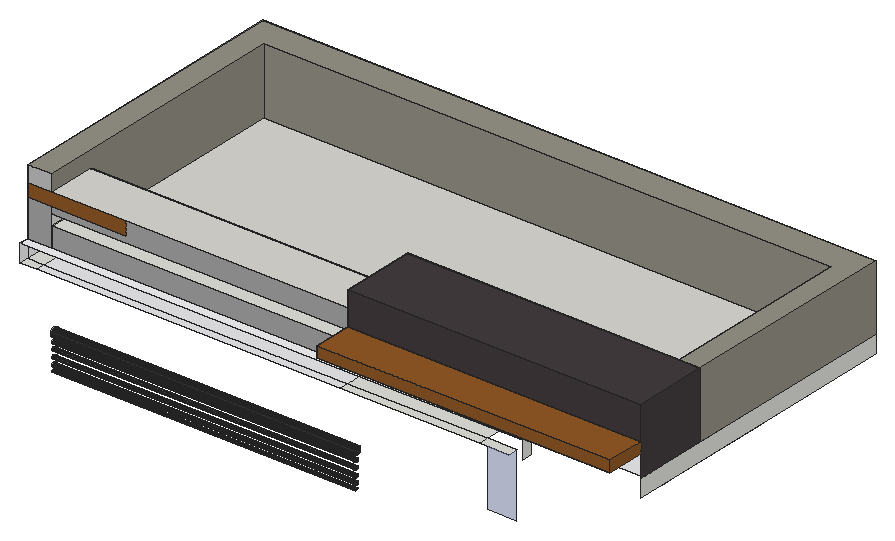
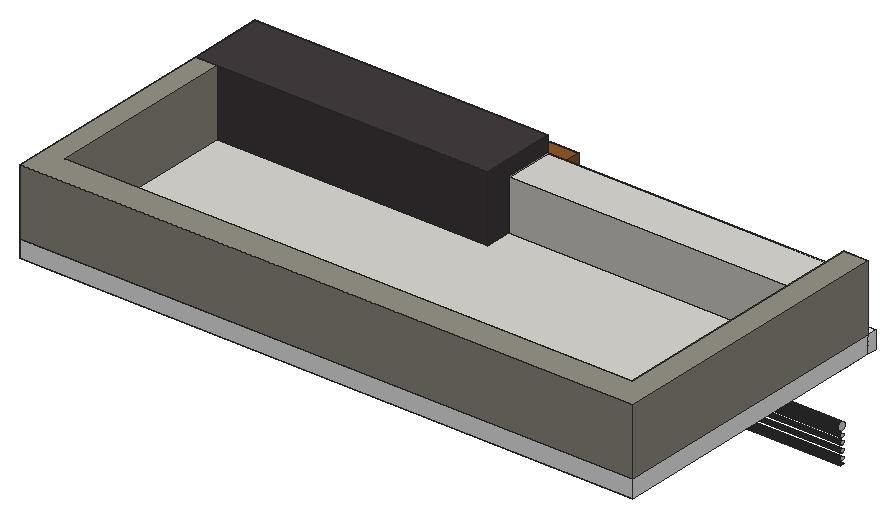
# SketchUp Ruby script. Lengths in inches.
U = 1.inch
M = Sketchup.active_model
def pt(a) = Geom::Point3d.new(a.map { |v| v * U })
def face(e, loops, mat)
  f = e.add_face(loops[0].map { |a| pt(a) })
  loops[1..].each { |l| e.add_face(l.map { |a| pt(a) }).erase! }
  f.material = f.back_material = mat if mat
  f
end
# faces: each face lists its corners as indices into pts; further lists are holes
def faces(e, pts, list, mat = nil) = list.each { |f| face(e, (f[0].is_a?(Array) ? f : [f]).map { |l| l.map { |i| pts[i] } }, mat) }
# xy, xz, yz: faces in a plane at the given z, y or x. An outline is a flat list of corners, or four numbers for a rectangle; further outlines are holes
def ring(l) = l.size == 4 ? [[l[0], l[1]], [l[2], l[1]], [l[2], l[3]], [l[0], l[3]]] : l.each_slice(2).to_a
def flat(e, list, mat, &to3) = list.each { |f| face(e, (f[0].is_a?(Array) ? f : [f]).map { |l| ring(l).map { |u, v| to3.(u, v) } }, mat) }
def xy(e, z, list, mat = nil) = flat(e, list, mat) { |x, y| [x, y, z] }
def xz(e, y, list, mat = nil) = flat(e, list, mat) { |x, z| [x, y, z] }
def yz(e, x, list, mat = nil) = flat(e, list, mat) { |y, z| [x, y, z] }
def lines(e, pts, list) = list.each { |a, b| e.add_line(pt(pts[a]), pt(pts[b])) }
# prism: a flat outline (further loops are holes) pulled along v
def prism(e, loops, v, mat = nil)
  f = face(e, loops, mat); d = Geom::Vector3d.new(v.map { |x| x * U })
  f.pushpull(f.normal.samedirection?(d) ? d.length : -d.length)
end
def box(e, o, s, mat = nil) = prism(e, [[o, [o[0] + s[0], o[1], o[2]], [o[0] + s[0], o[1] + s[1], o[2]], [o[0], o[1] + s[1], o[2]]]], [0, 0, s[2]], mat)
def at(x, y, z, deg = 0) = Geom::Transformation.translation(pt([x, y, z])) * Geom::Transformation.rotation(ORIGIN, Z_AXIS, deg.degrees)
def axes(o, x, y, z) = Geom::Transformation.new([*x, 0, *y, 0, *z, 0, *pt(o).to_a, 1])
def part(name) = M.definitions.add(name)
# library, detail: a bought-in or finely detailed component or shape, given as its bounding box
def library(name, o, s) = part(name).tap { |d| box(d.entities, o, s) }
def detail(e, o, s) = box(e.add_group.entities, o, s)
def put(e, d, t, mat = nil) = e.add_instance(d, t).tap { |i| i.material = mat if mat }
def group(e, t, mat = nil) = e.add_group.tap { |g| g.transformation = t; g.material = mat if mat }.entities
root = M.entities
M.materials.add("[Asphalt New]").color = [67, 60, 62]
M.materials.add("[Blinds Vertical Pattern]").color = [245, 245, 247]
M.materials.add("[Blinds Vertical Pattern]2").color = [234, 234, 237]
M.materials.add("[Blinds Vertical Pattern]3").color = [247, 247, 249]
M.materials.add("[Color M02]").color = [198, 198, 198]
M.materials.add("[Color M03]").color = [170, 170, 170]
M.materials.add("[Color M06]").color = [86, 86, 86]
M.materials.add("[Color M07]").color = [58, 58, 58]
M.materials.add("[Formica Graystone]1").color = [149, 146, 135]
M.materials.add("[Terrazzo Tile Light]").color = [219, 217, 210]
M.materials.add("[Translucent Glass Sky Reflection]").color = [126, 138, 183]
M.materials["[Translucent Glass Sky Reflection]"].alpha = 0.52
M.materials.add("[Wood Floor Parquet]").color = [145, 89, 39]
xy(root,782.625,[[64.24,456.35,65.12,456.36,65.97,456.59,66.73,457.03,67.35,457.66,67.79,458.43,68.01,459.28,68.01,460.16,67.77,461.01,67.33,461.77,66.7,462.39,65.9375,462.83,65.09,463.05,64.21,463.05,63.36,462.8125,62.6,462.37,61.98,461.74,61.54,460.98,61.31,460.125,61.32,459.24,61.55,458.39,62,457.63,62.62,457.01,63.39,456.58]])
xy(root,782.97,[[231.18,456.35,232.06,456.36,232.91,456.59,233.67,457.03,234.29,457.66,234.73,458.43,234.95,459.28,234.94,460.16,234.71,461.01,234.27,461.77,233.64,462.39,232.875,462.83,232.02,463.05,231.14,463.05,230.29,462.8125,229.53,462.37,228.91,461.74,228.48,460.98,228.25,460.125,228.26,459.24,228.49,458.39,228.93,457.63,229.56,457.01,230.32,456.58],[316.36,456.35,317.25,456.36,318.1,456.59,318.86,457.03,319.48,457.66,319.91,458.43,320.14,459.28,320.13,460.16,319.9,461.01,319.46,461.77,318.83,462.39,318.0625,462.83,317.21,463.05,316.33,463.05,315.48,462.8125,314.72,462.37,314.1,461.74,313.66,460.98,313.44,460.125,313.44,459.24,313.68,458.39,314.12,457.63,314.75,457.01,315.51,456.58]])
xy(root,784.2,[[408.8,456.35,409.68,456.36,410.53,456.59,411.29,457.03,411.91,457.66,412.35,458.43,412.57,459.28,412.57,460.16,412.34,461.01,411.89,461.77,411.27,462.39,410.5,462.83,409.65,463.05,408.77,463.05,407.92,462.8125,407.16,462.37,406.54,461.74,406.1,460.98,405.88,460.125,405.88,459.24,406.11,458.39,406.56,457.63,407.18,457.01,407.95,456.58]])
xy(root,785.43,[[137.99,456.35,138.87,456.36,139.72,456.59,140.48,457.03,141.1,457.66,141.54,458.43,141.76,459.28,141.76,460.16,141.52,461.01,141.08,461.77,140.45,462.39,139.6875,462.83,138.84,463.05,137.96,463.05,137.11,462.8125,136.35,462.37,135.73,461.74,135.29,460.98,135.06,460.125,135.07,459.24,135.3,458.39,135.75,457.63,136.37,457.01,137.14,456.58]])
xy(root,828.25,[[111.4,617.07,693.46,637.38]])
xy(root,861.625,[[36.42,435.375,56.39,446.5625],[415.32,435.375,580.71,446.5625],[580.71,435.375,615.19,446.5625],[36.42,446.5625,56.39,480.02],[415.32,446.5625,580.71,480.02],
  [36.42,480.02,56.39,499.99],[741.77,480.02,761.74,499.99],[36.42,499.99,56.39,617.07],[741.77,499.99,761.74,617.07],[36.42,617.07,56.39,637.38],
  [56.39,617.07,741.77,637.38],[741.77,617.07,761.74,637.38],[36.42,637.38,56.39,774.78],[56.39,637.38,741.77,774.78],[741.77,637.38,761.74,794.75],
  [36.42,774.78,741.77,794.75]])
xy(root,861.625,[[56.39,435.375,415.32,446.5625],[56.39,446.5625,56.39,617.07,741.77,617.07,741.77,480.02,415.32,480.02,415.32,446.5625]],"[Blinds Vertical Pattern]2")
xy(root,882.375,[[36.42,446.5625,36.42,794.75,761.74,794.75,761.74,534.9375,736.11,534.9375,736.11,759.5625,65.36,759.5625,65.36,446.5625],[65.36,446.5625,415.32,481.84],[65.36,481.84,415.32,504.47]])
xy(root,882.375,[[36.42,435.375,415.32,446.5625],[415.32,435.375,631.7,446.5625]],"[Blinds Vertical Pattern]")
xy(root,882.375,[[65.36,504.47,415.32,504.47,415.32,534.9375,736.11,534.9375,736.11,759.5625,65.36,759.5625]],"[Terrazzo Tile Light]")
xy(root,905.75,[[65.36,446.5625,415.32,481.84]])
xy(root,908.98,[[715.96,423.625,761.74,446.5625]])
xy(root,908.98,[[415.32,401.3125,415.32,446.5625,715.96,446.5625,715.96,423.625,761.74,423.625,761.74,401.3125]],"[Wood Floor Parquet]")
xy(root,918.49,[[65.36,446.5625,415.32,481.84]])
xy(root,921.875,[[415.32,401.3125,761.74,446.5625]],"[Wood Floor Parquet]")
xy(root,941.4375,[[65.36,446.5625,415.32,504.47]],"[Terrazzo Tile Light]")
xy(root,960.8125,[[415.32,446.5625,761.74,534.9375]],"[Asphalt New]")
xy(root,960.8125,[[36.42,446.5625,65.36,446.5625,65.36,759.5625,736.11,759.5625,736.11,534.9375,761.74,534.9375,761.74,794.75,36.42,794.75]],"[Formica Graystone]1")
xz(root,401.3125,[[415.32,908.98,761.74,921.875]],"[Wood Floor Parquet]")
xz(root,446.5625,[[415.32,908.98,761.74,921.875]])
xz(root,446.5625,[[415.32,921.875,761.74,960.8125]],"[Asphalt New]")
xz(root,446.5625,[[36.42,941.4375,65.36,960.8125]],"[Color M02]")
xz(root,446.5625,[[36.42,882.375,65.36,926.04],[65.36,882.375,415.32,905.75],[65.36,918.49,415.32,918.49,415.32,941.4375,152.8,941.4375,152.8,926.04,65.36,926.04]],"[Color M03]")
xz(root,446.5625,[[580.71,785.52,615.19,861.625]],"[Translucent Glass Sky Reflection]")
xz(root,446.5625,[[36.42,926.04,152.8,941.4375]],"[Wood Floor Parquet]")
xz(root,481.84,[[65.36,882.375,415.32,905.75]])
xz(root,481.84,[[65.36,905.75,415.32,918.49]],"[Blinds Vertical Pattern]")
xz(root,504.47,[[65.36,882.375,415.32,941.4375]],"[Terrazzo Tile Light]")
xz(root,534.9375,[[736.11,882.375,761.74,960.8125]])
xz(root,534.9375,[[415.32,882.375,736.11,960.8125]],"[Asphalt New]")
xz(root,759.5625,[[65.36,882.375,736.11,960.8125]],"[Formica Graystone]1")
xz(root,794.75,[[36.42,861.625,761.74,882.375]],"[Blinds Vertical Pattern]3")
xz(root,794.75,[[36.42,882.375,761.74,960.8125]],"[Formica Graystone]1")
yz(root,36.42,[[435.375,861.625,446.5625,882.375]],"[Blinds Vertical Pattern]")
yz(root,36.42,[[446.5625,861.625,794.75,882.375]],"[Blinds Vertical Pattern]3")
yz(root,36.42,[[446.5625,882.375,794.75,960.8125]],"[Formica Graystone]1")
yz(root,56.39,[[459.98,747.97,459.46,748.04,458.98,748.24,458.57,748.56,458.25,748.97,458.05,749.46,457.98,749.97,458.05,750.49,458.25,750.97,458.57,751.39,458.98,751.71,459.46,751.9,459.98,751.97,460.5,751.9,460.98,751.71,461.39,751.39,461.71,750.97,461.91,750.49,461.98,749.97,461.91,749.46,461.71,748.97,461.39,748.56,460.98,748.24,460.5,748.04],[459.98,756.16,459.46,756.23,458.98,756.43,458.57,756.75,458.25,757.16,458.05,757.64,457.98,758.16,458.05,758.68,458.25,759.16,458.57,759.57,458.98,759.89,459.46,760.09,459.98,760.16,460.5,760.09,460.98,759.89,461.39,759.57,461.71,759.16,461.91,758.68,461.98,758.16,461.91,757.64,461.71,757.16,461.39,756.75,460.98,756.43,460.5,756.23],[459.98,764.6,459.46,764.67,458.98,764.87,458.57,765.18,458.25,765.6,458.05,766.08,457.98,766.6,458.05,767.12,458.25,767.6,458.57,768.01,458.98,768.33,459.46,768.53,459.98,768.6,460.5,768.53,460.98,768.33,461.39,768.01,461.71,767.6,461.91,767.12,461.98,766.6,461.91,766.08,461.71,765.6,461.39,765.18,460.98,764.87,460.5,764.67],[459.98,772.35,459.46,772.42,458.98,772.62,458.57,772.93,458.25,773.35,458.05,773.83,457.98,774.35,458.05,774.87,458.25,775.35,458.57,775.76,458.98,776.08,459.46,776.28,459.98,776.35,460.5,776.28,460.98,776.08,461.39,775.76,461.71,775.35,461.91,774.87,461.98,774.35,461.91,773.83,461.71,773.35,461.39,772.93,460.98,772.62,460.5,772.42],[460.55,779.45,459.32,779.61,458.18,780.09,457.2,780.84,456.44,781.83,455.97,782.97,455.8,784.2,455.97,785.43,456.44,786.58,457.2,787.56,458.18,788.31,459.32,788.79,460.55,788.95,461.78,788.79,462.93,788.31,463.91,787.56,464.67,786.58,465.14,785.43,465.3,784.2,465.14,782.97,464.67,781.83,463.91,780.84,462.93,780.09,461.78,779.61]])
yz(root,65.36,[[446.5625,882.375,481.84,905.75],[446.5625,905.75,481.84,918.49]])
yz(root,65.36,[[504.47,882.375,759.5625,882.375,759.5625,960.8125,446.5625,960.8125,446.5625,941.4375,504.47,941.4375]],"[Formica Graystone]1")
yz(root,415.32,[[446.5625,882.375,481.84,905.75],[481.84,882.375,481.84,918.49,446.5625,918.49,446.5625,941.4375,504.47,941.4375,504.47,882.375]])
yz(root,415.32,[[504.47,882.375,504.47,941.4375,446.5625,941.4375,446.5625,960.8125,534.9375,960.8125,534.9375,882.375],[446.5625,905.75,481.84,918.49]],"[Asphalt New]")
yz(root,415.32,[[401.3125,908.98,446.5625,921.875]],"[Wood Floor Parquet]")
yz(root,631.7,[[435.375,861.625,446.5625,882.375]])
yz(root,736.11,[[534.9375,882.375,759.5625,960.8125]],"[Formica Graystone]1")
yz(root,761.74,[[446.5625,861.625,794.75,882.375]])
yz(root,761.74,[[446.5625,882.375,534.9375,960.8125]],"[Asphalt New]")
yz(root,761.74,[[534.9375,882.375,794.75,960.8125]],"[Formica Graystone]1")
yz(root,761.74,[[401.3125,908.98,446.5625,921.875]],"[Wood Floor Parquet]")
p = [[56.39,458.25,743.66],[56.39,458.05,743.18],[415.32,458.05,743.18],[415.32,458.25,743.66],[56.39,461.91,743.18],[56.39,461.71,743.66],
  [415.32,461.71,743.66],[415.32,461.91,743.18],[56.39,458.57,744.07],[415.32,458.57,744.07],[56.39,461.39,744.07],[415.32,461.39,744.07],
  [56.39,458.98,744.39],[415.32,458.98,744.39],[56.39,460.98,744.39],[415.32,460.98,744.39],[56.39,459.46,744.59],[415.32,459.46,744.59],
  [56.39,460.5,744.59],[415.32,460.5,744.59],[56.39,459.98,744.66],[415.32,459.98,744.66],[56.39,458.98,748.24],[56.39,459.46,748.04],
  [415.32,459.46,748.04],[415.32,458.98,748.24],[56.39,459.98,747.97],[415.32,459.98,747.97],[56.39,460.5,748.04],[415.32,460.5,748.04],
  [56.39,460.98,748.24],[415.32,460.98,748.24],[56.39,458.57,748.56],[415.32,458.57,748.56],[56.39,461.39,748.56],[415.32,461.39,748.56],
  [56.39,458.25,748.97],[415.32,458.25,748.97],[56.39,461.71,748.97],[415.32,461.71,748.97],[56.39,458.05,749.46],[415.32,458.05,749.46],
  [56.39,461.91,749.46],[415.32,461.91,749.46],[56.39,457.98,749.97],[415.32,457.98,749.97],[56.39,461.98,749.97],[415.32,461.98,749.97],
  [56.39,458.05,750.49],[415.32,458.05,750.49],[56.39,461.91,750.49],[415.32,461.91,750.49],[56.39,458.25,750.97],[415.32,458.25,750.97],
  [56.39,461.71,750.97],[415.32,461.71,750.97],[56.39,458.57,751.39],[415.32,458.57,751.39],[56.39,461.39,751.39],[415.32,461.39,751.39],
  [56.39,458.98,751.71],[415.32,458.98,751.71],[56.39,460.98,751.71],[415.32,460.98,751.71],[56.39,459.46,751.9],[415.32,459.46,751.9],
  [56.39,460.5,751.9],[415.32,460.5,751.9],[56.39,459.98,751.97],[415.32,459.98,751.97],[56.39,458.98,756.43],[56.39,459.46,756.23],
  [415.32,459.46,756.23],[415.32,458.98,756.43],[56.39,459.98,756.16],[415.32,459.98,756.16],[56.39,460.5,756.23],[415.32,460.5,756.23],
  [56.39,460.98,756.43],[415.32,460.98,756.43],[56.39,458.57,756.75],[415.32,458.57,756.75],[56.39,461.39,756.75],[415.32,461.39,756.75],
  [56.39,458.25,757.16],[415.32,458.25,757.16],[56.39,461.71,757.16],[415.32,461.71,757.16],[56.39,458.05,757.64],[415.32,458.05,757.64],
  [56.39,461.91,757.64],[415.32,461.91,757.64],[56.39,457.98,758.16],[415.32,457.98,758.16],[56.39,461.98,758.16],[415.32,461.98,758.16],
  [56.39,458.05,758.68],[415.32,458.05,758.68],[56.39,461.91,758.68],[415.32,461.91,758.68],[56.39,458.25,759.16],[415.32,458.25,759.16],
  [56.39,461.71,759.16],[415.32,461.71,759.16],[56.39,458.57,759.57],[415.32,458.57,759.57],[56.39,461.39,759.57],[415.32,461.39,759.57],
  [56.39,458.98,759.89],[415.32,458.98,759.89],[56.39,460.98,759.89],[415.32,460.98,759.89],[56.39,459.46,760.09],[415.32,459.46,760.09],
  [56.39,460.5,760.09],[415.32,460.5,760.09],[56.39,459.98,760.16],[415.32,459.98,760.16],[56.39,459.46,764.67],[56.39,459.98,764.6],
  [415.32,459.98,764.6],[415.32,459.46,764.67],[56.39,460.5,764.67],[415.32,460.5,764.67],[56.39,458.98,764.87],[415.32,458.98,764.87],
  [56.39,460.98,764.87],[415.32,460.98,764.87],[56.39,458.57,765.18],[415.32,458.57,765.18],[56.39,461.39,765.18],[415.32,461.39,765.18],
  [56.39,458.25,765.6],[415.32,458.25,765.6],[56.39,461.71,765.6],[415.32,461.71,765.6],[56.39,458.05,766.08],[415.32,458.05,766.08],
  [56.39,461.91,766.08],[415.32,461.91,766.08],[56.39,457.98,766.6],[415.32,457.98,766.6],[56.39,461.98,766.6],[415.32,461.98,766.6],
  [56.39,458.05,767.12],[415.32,458.05,767.12],[56.39,461.91,767.12],[415.32,461.91,767.12],[56.39,458.25,767.6],[415.32,458.25,767.6],
  [56.39,461.71,767.6],[415.32,461.71,767.6],[56.39,458.57,768.01],[415.32,458.57,768.01],[56.39,461.39,768.01],[415.32,461.39,768.01],
  [56.39,458.98,768.33],[415.32,458.98,768.33],[56.39,460.98,768.33],[415.32,460.98,768.33],[56.39,459.46,768.53],[415.32,459.46,768.53],
  [56.39,460.5,768.53],[415.32,460.5,768.53],[56.39,459.98,768.6],[415.32,459.98,768.6],[56.39,459.46,772.42],[56.39,459.98,772.35],
  [415.32,459.98,772.35],[415.32,459.46,772.42],[56.39,460.5,772.42],[415.32,460.5,772.42],[56.39,458.98,772.62],[415.32,458.98,772.62],
  [56.39,460.98,772.62],[415.32,460.98,772.62],[56.39,458.57,772.93],[415.32,458.57,772.93],[56.39,461.39,772.93],[415.32,461.39,772.93],
  [56.39,458.25,773.35],[415.32,458.25,773.35],[56.39,461.71,773.35],[415.32,461.71,773.35],[56.39,458.05,773.83],[415.32,458.05,773.83],
  [56.39,461.91,773.83],[415.32,461.91,773.83],[56.39,457.98,774.35],[415.32,457.98,774.35],[56.39,461.98,774.35],[415.32,461.98,774.35],
  [56.39,458.05,774.87],[415.32,458.05,774.87],[56.39,461.91,774.87],[415.32,461.91,774.87],[56.39,458.25,775.35],[415.32,458.25,775.35],
  [56.39,461.71,775.35],[415.32,461.71,775.35],[56.39,458.57,775.76],[415.32,458.57,775.76],[56.39,461.39,775.76],[415.32,461.39,775.76],
  [56.39,458.98,776.08],[415.32,458.98,776.08],[56.39,460.98,776.08],[415.32,460.98,776.08],[56.39,459.46,776.28],[415.32,459.46,776.28],
  [56.39,460.5,776.28],[415.32,460.5,776.28],[56.39,459.98,776.35],[415.32,459.98,776.35],[56.39,459.32,779.61],[56.39,460.55,779.45],
  [415.32,460.55,779.45],[415.32,459.32,779.61],[56.39,461.78,779.61],[415.32,461.78,779.61],[56.39,458.18,780.09],[415.32,458.18,780.09],
  [56.39,462.93,780.09],[415.32,462.93,780.09],[56.39,457.2,780.84],[415.32,457.2,780.84],[56.39,463.91,780.84],[415.32,463.91,780.84],
  [56.39,456.44,781.83],[415.32,456.44,781.83],[56.39,464.67,781.83],[415.32,464.67,781.83],[56.39,455.97,782.97],[415.32,455.97,782.97],
  [56.39,465.14,782.97],[415.32,465.14,782.97],[56.39,455.8,784.2],[415.32,455.8,784.2],[56.39,465.3,784.2],[415.32,465.3,784.2],
  [56.39,455.97,785.43],[415.32,455.97,785.43],[56.39,465.14,785.43],[415.32,465.14,785.43],[56.39,456.44,786.58],[415.32,456.44,786.58],
  [56.39,464.67,786.58],[415.32,464.67,786.58],[56.39,457.2,787.56],[415.32,457.2,787.56],[56.39,463.91,787.56],[415.32,463.91,787.56],
  [56.39,458.18,788.31],[415.32,458.18,788.31],[56.39,462.93,788.31],[415.32,462.93,788.31],[56.39,459.32,788.79],[415.32,459.32,788.79],
  [56.39,461.78,788.79],[415.32,461.78,788.79],[56.39,460.55,788.95],[415.32,460.55,788.95]]
faces(root,p,[[0,1,2,3],[4,5,6,7],[8,0,3,9],[5,10,11,6],[12,8,9,13],[10,14,15,11],[16,12,13,17],[14,18,19,15],
  [20,16,17,21],[18,20,21,19],[22,23,24,25],[23,26,27,24],[26,28,29,27],[28,30,31,29],[32,22,25,33],[30,34,35,31],
  [36,32,33,37],[34,38,39,35],[40,36,37,41],[38,42,43,39],[44,40,41,45],[42,46,47,43],[48,44,45,49],[46,50,51,47],
  [52,48,49,53],[50,54,55,51],[56,52,53,57],[54,58,59,55],[60,56,57,61],[58,62,63,59],[64,60,61,65],[62,66,67,63],
  [68,64,65,69],[66,68,69,67],[70,71,72,73],[71,74,75,72],[74,76,77,75],[76,78,79,77],[80,70,73,81],[78,82,83,79],
  [84,80,81,85],[82,86,87,83],[88,84,85,89],[86,90,91,87],[92,88,89,93],[90,94,95,91],[96,92,93,97],[94,98,99,95],
  [100,96,97,101],[98,102,103,99],[104,100,101,105],[102,106,107,103],[108,104,105,109],[106,110,111,107],[112,108,109,113],[110,114,115,111],
  [116,112,113,117],[114,116,117,115],[118,119,120,121],[119,122,123,120],[124,118,121,125],[122,126,127,123],[128,124,125,129],[126,130,131,127],
  [132,128,129,133],[130,134,135,131],[136,132,133,137],[134,138,139,135],[140,136,137,141],[138,142,143,139],[144,140,141,145],[142,146,147,143],
  [148,144,145,149],[146,150,151,147],[152,148,149,153],[150,154,155,151],[156,152,153,157],[154,158,159,155],[160,156,157,161],[158,162,163,159],
  [164,160,161,165],[162,164,165,163],[166,167,168,169],[167,170,171,168],[172,166,169,173],[170,174,175,171],[176,172,173,177],[174,178,179,175],
  [180,176,177,181],[178,182,183,179],[184,180,181,185],[182,186,187,183],[188,184,185,189],[186,190,191,187],[192,188,189,193],[190,194,195,191],
  [196,192,193,197],[194,198,199,195],[200,196,197,201],[198,202,203,199],[204,200,201,205],[202,206,207,203],[208,204,205,209],[206,210,211,207],
  [212,208,209,213],[210,212,213,211]],"[Color M06]")
faces(root,p,[[214,215,216,217],[215,218,219,216],[220,214,217,221],[218,222,223,219],[224,220,221,225],[222,226,227,223],[228,224,225,229],[226,230,231,227],
  [232,228,229,233],[230,234,235,231],[236,232,233,237],[234,238,239,235],[240,236,237,241],[238,242,243,239],[244,240,241,245],[242,246,247,243],
  [248,244,245,249],[246,250,251,247],[252,248,249,253],[250,254,255,251],[256,252,253,257],[254,258,259,255],[260,256,257,261],[258,260,261,259]],"[Color M07]")
